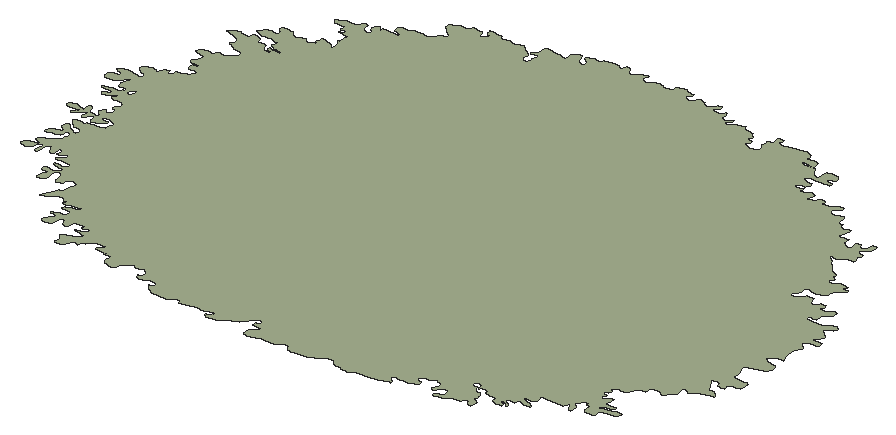
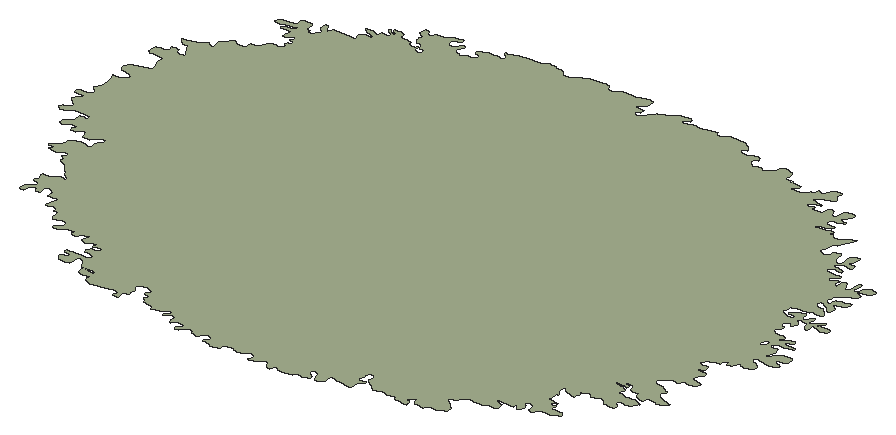
# SketchUp Ruby script. Lengths in inches.
U = 1.inch
M = Sketchup.active_model
def pt(a) = Geom::Point3d.new(a.map { |v| v * U })
def face(e, loops, mat)
  f = e.add_face(loops[0].map { |a| pt(a) })
  loops[1..].each { |l| e.add_face(l.map { |a| pt(a) }).erase! }
  f.material = f.back_material = mat if mat
  f
end
# faces: each face lists its corners as indices into pts; further lists are holes
def faces(e, pts, list, mat = nil) = list.each { |f| face(e, (f[0].is_a?(Array) ? f : [f]).map { |l| l.map { |i| pts[i] } }, mat) }
# xy, xz, yz: faces in a plane at the given z, y or x. An outline is a flat list of corners, or four numbers for a rectangle; further outlines are holes
def ring(l) = l.size == 4 ? [[l[0], l[1]], [l[2], l[1]], [l[2], l[3]], [l[0], l[3]]] : l.each_slice(2).to_a
def flat(e, list, mat, &to3) = list.each { |f| face(e, (f[0].is_a?(Array) ? f : [f]).map { |l| ring(l).map { |u, v| to3.(u, v) } }, mat) }
def xy(e, z, list, mat = nil) = flat(e, list, mat) { |x, y| [x, y, z] }
def xz(e, y, list, mat = nil) = flat(e, list, mat) { |x, z| [x, y, z] }
def yz(e, x, list, mat = nil) = flat(e, list, mat) { |y, z| [x, y, z] }
def lines(e, pts, list) = list.each { |a, b| e.add_line(pt(pts[a]), pt(pts[b])) }
# prism: a flat outline (further loops are holes) pulled along v
def prism(e, loops, v, mat = nil)
  f = face(e, loops, mat); d = Geom::Vector3d.new(v.map { |x| x * U })
  f.pushpull(f.normal.samedirection?(d) ? d.length : -d.length)
end
def box(e, o, s, mat = nil) = prism(e, [[o, [o[0] + s[0], o[1], o[2]], [o[0] + s[0], o[1] + s[1], o[2]], [o[0], o[1] + s[1], o[2]]]], [0, 0, s[2]], mat)
def at(x, y, z, deg = 0) = Geom::Transformation.translation(pt([x, y, z])) * Geom::Transformation.rotation(ORIGIN, Z_AXIS, deg.degrees)
def axes(o, x, y, z) = Geom::Transformation.new([*x, 0, *y, 0, *z, 0, *pt(o).to_a, 1])
def part(name) = M.definitions.add(name)
# library, detail: a bought-in or finely detailed component or shape, given as its bounding box
def library(name, o, s) = part(name).tap { |d| box(d.entities, o, s) }
def detail(e, o, s) = box(e.add_group.entities, o, s)
def put(e, d, t, mat = nil) = e.add_instance(d, t).tap { |i| i.material = mat if mat }
def group(e, t, mat = nil) = e.add_group.tap { |g| g.transformation = t; g.material = mat if mat }.entities
root = M.entities
M.materials.add("Boxwoodplan").color = [166, 177, 144]
xy(root,9,[[[264.536,68.149,264.425,68.153,264.33,68.178,264.274,68.234,264.272,68.337,264.298,68.401,264.362,68.464,264.411,68.528,264.469,68.625,264.283,68.655,264.193,68.664,264.213,68.752,264.299,68.81,264.33,68.82,264.325,68.865,264.236,68.897,264.12,68.856,264.023,68.726,263.88,68.571,263.719,68.484,263.614,68.461,263.553,68.436,263.537,68.393,263.393,68.301,263.199,68.271,263.11,68.279,263.03,68.326,263.03,68.347,263.075,68.378,263.166,68.456,263.234,68.503,263.145,68.517,263.032,68.5,262.912,68.455,262.816,68.464,262.719,68.474,262.622,68.466,262.495,68.422,262.295,68.376,262.206,68.369,262.168,68.462,262.16,68.484,262.093,68.492,262.004,68.474,261.835,68.356,261.636,68.347,261.405,68.373,261.238,68.466,261.097,68.63,261.28,68.722,261.18,68.775,261.044,68.792,260.918,68.769,260.846,68.716,260.765,68.692,260.649,68.757,260.607,68.825,260.695,68.866,260.722,68.927,260.726,68.977,260.685,69.029,260.613,69.105,260.527,69.137,260.44,69.084,260.374,69.058,260.318,69.1,260.301,69.123,260.277,69.141,260.248,69.131,260.169,69.077,260.097,69.029,260.021,68.943,260.009,68.81,259.938,68.768,259.888,68.743,259.828,68.745,259.729,68.765,259.642,68.813,259.598,68.881,259.59,68.971,259.599,69.037,259.612,69.059,259.593,69.1,259.379,69.119,259.447,69.155,259.421,69.156,259.328,69.15,259.159,69.166,259.082,69.192,259.064,69.226,259.079,69.244,259.204,69.333,259.202,69.39,259.117,69.413,258.958,69.409,258.827,69.339,258.73,69.253,258.655,69.218,258.608,69.192,258.607,69.173,258.643,69.121,258.627,69.066,258.557,69.101,258.493,69.14,258.432,69.092,258.41,69.037,258.378,68.923,258.331,68.875,258.258,68.841,258.167,68.836,258.097,68.861,258.078,68.894,258.085,68.912,258.106,68.952,258.128,69.011,258.097,69.068,257.996,69.169,258.11,69.249,258.171,69.289,258.251,69.304,258.318,69.335,258.373,69.389,258.458,69.496,258.386,69.522,258.307,69.53,258.174,69.55,258.136,69.585,258.143,69.604,258.218,69.639,258.38,69.677,258.422,69.728,258.417,69.768,258.391,69.783,258.241,69.731,258.195,69.752,258.196,69.771,258.219,69.834,258.058,69.845,257.977,69.853,257.923,69.845,257.916,69.826,257.9,69.729,257.885,69.662,257.843,69.611,257.796,69.598,257.777,69.613,257.718,69.659,257.673,69.777,257.634,69.803,257.607,69.804,257.553,69.796,257.546,69.777,257.544,69.661,257.49,69.543,257.429,69.469,257.349,69.439,257.27,69.442,257.224,69.467,257.191,69.526,257.191,69.583,257.245,69.697,257.359,69.804,257.379,69.822,257.366,69.843,257.339,69.848,257.259,69.866,257.178,69.879,257.151,69.895,257.158,69.914,257.178,69.933,257.327,70.001,257.489,70.025,257.531,70.127,257.505,70.188,257.457,70.21,257.43,70.206,257.267,70.188,257.226,70.219,257.233,70.239,257.26,70.299,257.418,70.353,257.59,70.423,257.638,70.462,257.625,70.483,257.529,70.456,257.357,70.437,257.213,70.392,257.124,70.405,257.097,70.411,257.103,70.431,257.124,70.446,257.179,70.49,257.151,70.527,257.124,70.523,257.041,70.531,256.986,70.579,256.972,70.621,256.945,70.617,256.862,70.594,256.705,70.508,256.556,70.432,256.482,70.4,256.427,70.412,256.44,70.432,256.459,70.472,256.486,70.489,256.51,70.569,256.56,70.67,256.592,70.778,256.643,70.832,256.717,70.871,256.76,70.992,256.782,71.132,256.802,71.246,256.798,71.305,256.753,71.341,256.672,71.354,256.586,71.354,256.512,71.33,256.503,71.265,256.503,71.203,256.47,71.144,256.382,71.107,256.325,71.116,256.287,71.175,256.276,71.236,256.25,71.357,256.245,71.419,256.204,71.473,256.177,71.495,256.139,71.51,256.081,71.499,256.046,71.479,256.044,71.448,256.036,71.386,256.039,71.249,256.064,71.187,256.056,71.123,256.005,71.058,255.957,71.03,255.919,71.018,255.881,71.023,255.839,71.031,255.821,71.058,255.817,71.186,255.838,71.243,255.884,71.296,255.899,71.326,255.891,71.354,255.834,71.359,255.752,71.366,255.715,71.381,255.692,71.41,255.689,71.472,255.704,71.503,255.739,71.519,255.911,71.491,255.99,71.516,256.039,71.546,256.1,71.593,256.113,71.656,256.09,71.682,256.046,71.683,255.969,71.69,255.877,71.701,255.776,71.737,255.757,71.766,255.763,71.78,255.782,71.783,255.842,71.795,256.017,71.781,256.107,71.806,256.119,71.864,256.093,71.926,256.021,71.966,255.943,71.972,255.829,71.966,255.729,71.94,255.646,71.958,255.642,71.988,255.663,72.016,255.709,72.073,255.775,72.13,255.828,72.21,255.82,72.244,255.775,72.261,255.71,72.259,255.592,72.159,255.553,72.161,255.518,72.181,255.54,72.24,255.556,72.307,255.513,72.369,255.473,72.386,255.453,72.387,255.447,72.372,255.451,72.326,255.449,72.184,255.408,72.122,255.368,72.127,255.333,72.151,255.235,72.282,255.211,72.347,255.186,72.374,255.171,72.363,255.116,72.3125,255.08,72.254,255.1,72.123,255.105,72.056,255.085,71.991,255.035,71.982,255.001,71.998,254.991,72.042,255.011,72.174,255.02,72.252,255.02,72.29,255.005,72.302,254.99,72.291,254.911,72.257,254.871,72.202,254.862,72.139,254.823,72.097,254.686,72.006,254.646,71.997,254.602,72.006,254.522,72.046,254.502,72.076,254.506,72.109,254.539,72.17,254.637,72.256,254.726,72.283,254.816,72.283,254.911,72.287,254.85,72.338,254.699,72.424,254.683,72.485,254.735,72.523,254.827,72.593,254.946,72.654,255.064,72.729,255.1,72.742,255.126,72.766,255.152,72.809,255.155,72.901,255.1875,73.022,255.189,73.084,255.168,73.105,255.146,73.114,255.083,73.129,255.05,73.124,255.046,73.108,255.058,73.015,255.016,72.954,254.968,72.918,254.891,72.89,254.82,72.878,254.659,72.853,254.624,72.858,254.611,72.872,254.611,72.88,254.62,72.92,254.637,72.967,254.679,73.014,254.748,73.061,254.807,73.083,254.865,73.085,254.904,73.087,254.924,73.095,254.947,73.116,254.942,73.14,254.888,73.171,254.82,73.227,254.788,73.284,254.784,73.351,254.797,73.401,254.849,73.446,254.875,73.451,254.886,73.445,254.906,73.431,254.949,73.37,254.998,73.324,255.126,73.246,255.2,73.212,255.235,73.196,255.255,73.204,255.279,73.226,255.286,73.242,255.297,73.283,255.282,73.34,255.239,73.386,255.207,73.409,255.173,73.421,255.113,73.421,255.039,73.424,254.996,73.466,254.91,73.538,254.851,73.589,254.812,73.636,254.813,73.665,254.837,73.691,254.893,73.718,254.928,73.723,254.969,73.719,255.03,73.699,255.091,73.697,255.127,73.704,255.161,73.745,255.21,73.777,255.27,73.784,255.34,73.783,255.494,73.791,255.634,73.811,255.667,73.828,255.668,73.846,255.662,73.888,255.65,73.932,255.662,73.976,255.691,74.08,255.678,74.103,255.655,74.116,255.599,74.146,255.545,74.183,255.473,74.211,255.399,74.214,255.349,74.204,255.328,74.19,255.303,74.138,255.308,74.117,255.319,74.113,255.343,74.108,255.494,74.096,255.52,74.091,255.525,74.082,255.516,74.066,255.476,74.026,255.431,73.983,255.366,73.947,255.304,73.904,255.232,73.868,255.195,73.872,255.175,73.883,255.15,73.92,255.143,74.015,255.126,74.04,255.144,74.054,255.15,74.097,255.145,74.107,255.133,74.108,255.118,74.106,255.092,74.103,255.06,74.096,255.042,74.084,254.961,73.989,254.929,73.934,254.898,73.911,254.875,73.914,254.849,73.935,254.841,73.952,254.834,73.992,254.863,74.077,254.868,74.122,254.859,74.149,254.839,74.156,254.801,74.147,254.781,74.134,254.735,74.084,254.613,73.977,254.577,73.952,254.551,73.947,254.514,73.954,254.502,73.971,254.593,74.077,254.656,74.122,254.67,74.148,254.669,74.165,254.661,74.172,254.649,74.168,254.634,74.162,254.603,74.151,254.519,74.127,254.352,74.109,254.279,74.116,254.231,74.141,254.209,74.168,254.208,74.185,254.225,74.237,254.273,74.283,254.333,74.3,254.404,74.304,254.478,74.286,254.606,74.243,254.692,74.217,254.703,74.22,254.703,74.239,254.694,74.259,254.669,74.306,254.668,74.362,254.675,74.427,254.687,74.457,254.704,74.469,254.753,74.432,254.792,74.383,254.819,74.337,254.829,74.275,254.841,74.223,254.856,74.195,254.879,74.195,255.014,74.177,255.087,74.163,255.122,74.16,255.14,74.174,255.155,74.222,255.1,74.264,255.042,74.328,255.024,74.355,255.024,74.372,255.058,74.48,255.088,74.503,255.115,74.508,255.13,74.497,255.139,74.479,255.168,74.434,255.179,74.409,255.191,74.411,255.213,74.423,255.292,74.501,255.309,74.547,255.31,74.599,255.296,74.631,255.275,74.643,255.212,74.666,255.172,74.685,255.164,74.706,255.18,74.756,255.236,74.793,255.27,74.815,255.283,74.835,255.291,74.889,255.289,74.936,255.194,75.011,255.05,75.034,254.988,75.05,254.953,75.033,254.925,75.034,254.856,75.051,254.837,75.078,254.846,75.102,254.972,75.204,254.966,75.237,254.944,75.252,254.899,75.244,254.871,75.235,254.744,75.174,254.704,75.127,254.655,75.083,254.586,75.068,254.558,75.069,254.511,75.121,254.539,75.146,254.557,75.185,254.588,75.208,254.682,75.239,254.727,75.269,254.716,75.3,254.703,75.303,254.693,75.296,254.667,75.289,254.628,75.292,254.493,75.304,254.346,75.332,254.322,75.347,254.328,75.366,254.353,75.395,254.566,75.455,254.629,75.454,254.69,75.438,254.75,75.41,254.777,75.412,254.783,75.422,254.832,75.5,254.856,75.515,254.862,75.534,254.862,75.602,254.852,75.613,254.838,75.61,254.78,75.611,254.723,75.604,254.676,75.587,254.652,75.595,254.631,75.616,254.606,75.649,254.586,75.737,254.597,75.826,254.627,75.868,254.633,75.9,254.646,75.942,254.684,75.964,254.679,76.01,254.657,76.046,254.568,76.023,254.55,75.989,254.551,75.969,254.554,75.906,254.474,75.859,254.333,75.765,254.177,75.72,254.093,75.745,254.051,75.798,254.042,75.924,254.17,76.009,254.253,76.023,254.297,76.047,254.32,76.081,254.319,76.101,254.233,76.132,254.16,76.158,254.098,76.214,254.133,76.268,254.209,76.297,254.305,76.331,254.37,76.33,254.549,76.287,254.641,76.265,254.726,76.269,254.777,76.289,254.783,76.309,254.767,76.375,254.706,76.427,254.661,76.434,254.549,76.505,254.502,76.547,254.488,76.583,254.481,76.637,254.481,76.664,254.494,76.679,254.536,76.714,254.587,76.729,254.701,76.76,254.732,76.77,254.772,76.77,254.822,76.765,254.835,76.753,254.85,76.723,254.864,76.709,254.874,76.709,254.902,76.712,254.918,76.724,254.939,76.774,254.967,76.807,254.983,76.83,254.986,76.855,255.002,76.88,255.022,76.892,255.07,76.904,255.109,76.896,255.13,76.853,255.135,76.801,255.151,76.774,255.172,76.774,255.214,76.816,255.239,76.858,255.254,76.962,255.269,76.987,255.301,76.994,255.333,76.994,255.352,76.982,255.373,76.96,255.405,76.959,255.458,76.981,255.502,77.027,255.516,77.051,255.505,77.065,255.565,77.063,255.594,77.066,255.61,77.085,255.615,77.134,255.649,77.174,255.683,77.22,255.629,77.263,255.562,77.292,255.525,77.291,255.492,77.28,255.45,77.269,255.408,77.275,255.386,77.291,255.365,77.314,255.342,77.417,255.355,77.442,255.36,77.459,255.371,77.462,255.475,77.483,255.521,77.491,255.539,77.502,255.529,77.506,255.444,77.534,255.378,77.546,255.349,77.539,255.314,77.539,255.278,77.54,255.242,77.552,255.204,77.602,255.186,77.631,255.186,77.662,255.201,77.683,255.23,77.698,255.261,77.717,255.27,77.744,255.326,77.856,255.332,77.909,255.325,77.936,255.285,77.947,255.207,77.973,255.034,78.02,254.998,78.038,254.981,78.062,255.017,78.116,255.061,78.151,255.107,78.178,255.162,78.198,255.214,78.207,255.267,78.204,255.322,78.18,255.377,78.182,255.404,78.186,255.417,78.207,255.434,78.248,255.472,78.284,255.492,78.302,255.518,78.304,255.587,78.287,255.649,78.276,255.676,78.273,255.699,78.288,255.786,78.355,255.873,78.421,255.927,78.517,255.923,78.562,255.882,78.598,255.765,78.636,255.639,78.667,255.553,78.739,255.495,78.774,255.426,78.795,255.399,78.807,255.385,78.828,255.407,78.874,255.455,78.916,255.453,79.001,255.403,79.079,255.273,79.136,254.985,79.232,254.964,79.266,255.036,79.33,255.157,79.382,255.262,79.386,255.319,79.373,255.364,79.347,255.412,79.337,255.465,79.345,255.526,79.357,255.555,79.388,255.57,79.467,255.587,79.502,255.641,79.501,255.698,79.491,255.746,79.471,255.813,79.412,255.837,79.377,255.851,79.337,255.852,79.269,255.859,79.264,255.867,79.269,255.894,79.282,255.945,79.288,256.034,79.29,256.114,79.254,256.148,79.19,256.173,79.112,256.243,79.067,256.283,79.054,256.301,79.054,256.328,79.063,256.423,79.069,256.44,79.074,256.42,79.091,256.357,79.114,256.305,79.119,256.267,79.137,256.248,79.172,256.245,79.184,256.249,79.204,256.263,79.211,256.298,79.211,256.34,79.204,256.446,79.176,256.561,79.171,256.613,79.179,256.631,79.181,256.658,79.193,256.613,79.223,256.572,79.233,256.486,79.247,256.428,79.261,256.387,79.264,256.365,79.268,256.34,79.282,256.288,79.309,256.241,79.335,256.219,79.367,256.229,79.423,256.258,79.462,256.299,79.491,256.259,79.522,256.204,79.537,256.161,79.54,256.106,79.548,256.075,79.574,256.057,79.611,256.043,79.62,256.014,79.619,255.899,79.591,255.846,79.577,255.797,79.578,255.75,79.581,255.7,79.598,255.652,79.615,255.612,79.622,255.569,79.646,255.526,79.669,255.551,79.682,255.553,79.689,255.564,79.729,255.58,79.765,255.606,79.802,255.637,79.834,255.681,79.859,255.734,79.881,255.779,79.893,255.885,79.887,255.962,79.881,255.996,79.877,256.006,79.877,256.006,79.89,255.998,79.932,255.977,79.976,255.941,80.015,255.898,80.046,255.865,80.092,255.867,80.116,255.878,80.136,255.925,80.166,255.978,80.189,256.004,80.189,256.03,80.183,256.084,80.167,256.152,80.162,256.199,80.147,256.223,80.134,256.241,80.115,256.285,80.074,256.324,80.04,256.369,80.008,256.425,79.995,256.479,80,256.524,80.029,256.556,80.065,256.605,80.103,256.631,80.103,256.653,80.088,256.694,80.047,256.741,80.013,256.869,80.038,256.943,80.057,256.985,80.085,256.99,80.105,256.969,80.121,256.918,80.143,256.908,80.166,256.916,80.189,256.932,80.233,256.939,80.293,256.943,80.318,256.966,80.334,256.993,80.336,257.023,80.327,257.065,80.308,257.199,80.268,257.26,80.246,257.299,80.213,257.326,80.173,257.341,80.15,257.348,80.142,257.357,80.146,257.365,80.151,257.398,80.196,257.404,80.231,257.394,80.334,257.372,80.382,257.348,80.417,257.313,80.456,257.303,80.485,257.314,80.497,257.325,80.494,257.347,80.496,257.346,80.504,257.351,80.527,257.344,80.569,257.329,80.725,257.331,80.802,257.216,80.821,257.119,80.824,257.057,80.832,257.039,80.839,257.025,80.849,257.038,80.859,257.151,80.901,257.185,80.93,257.184,80.943,257.161,80.967,257.125,80.971,257.072,80.96,257.024,80.938,257.007,80.938,256.992,80.965,257.019,81.048,257.021,81.088,257.02,81.102,256.996,81.123,256.907,81.105,256.794,81.108,256.685,81.124,256.624,81.205,256.622,81.232,256.66,81.269,256.756,81.323,256.805,81.349,256.859,81.355,256.984,81.352,257.075,81.356,257.135,81.365,257.175,81.403,257.215,81.438,257.223,81.481,257.249,81.52,257.305,81.533,257.342,81.528,257.385,81.494,257.396,81.408,257.403,81.319,257.427,81.277,257.482,81.251,257.574,81.231,257.629,81.254,257.647,81.295,257.624,81.338,257.577,81.375,257.521,81.462,257.557,81.541,257.631,81.623,257.65,81.626,257.674,81.596,257.693,81.548,257.767,81.466,257.795,81.44,257.786,81.495,257.768,81.59,257.824,81.607,257.885,81.601,258.012,81.598,258.125,81.595,258.247,81.577,258.265,81.577,258.253,81.606,258.202,81.648,258.072,81.7,258.034,81.709,258.011,81.754,258.013,81.845,258.048,81.89,258.097,81.916,258.213,81.921,258.31,81.93,258.405,81.997,258.531,82.001,258.647,81.991,258.743,81.972,258.864,81.965,258.907,82.011,258.921,82.058,258.963,82.152,259.052,82.206,259.172,82.264,259.184,82.28,259.167,82.313,259.127,82.351,259.019,82.433,258.951,82.506,258.893,82.548,258.836,82.59,258.867,82.597,258.866,82.61,258.861,82.631,258.85,82.699,258.853,82.729,258.888,82.764,258.971,82.804,259.054,82.841,259.092,82.847,259.148,82.845,259.235,82.836,259.259,82.828,259.282,82.83,259.314,82.863,259.366,82.938,259.402,82.952,259.459,82.955,259.561,82.95,259.657,82.918,259.689,82.897,259.718,82.855,259.719,82.784,259.722,82.756,259.727,82.734,259.75,82.724,259.803,82.734,259.848,82.764,259.91,82.818,259.935,82.841,259.956,82.853,259.969,82.87,259.885,82.917,259.846,82.932,259.803,82.976,259.778,83.055,259.779,83.086,259.837,83.103,260.029,83.074,260.126,83.059,260.161,83.045,260.161,82.999,260.171,82.971,260.231,82.967,260.335,82.982,260.437,82.995,260.479,82.991,260.526,82.977,260.553,82.954,260.578,82.953,260.603,82.962,260.747,82.991,260.788,83,260.84,83.007,260.876,83.003,260.921,82.977,260.951,82.906,260.977,82.882,261.022,82.864,261.062,82.853,261.102,82.828,261.154,82.773,261.208,82.716,261.195,82.639,261.188,82.565,261.202,82.535,261.233,82.504,261.26,82.481,261.307,82.473,261.344,82.47,261.388,82.5,261.401,82.532,261.402,82.573,261.39,82.647,261.427,82.807,261.416,82.836,261.398,82.849,261.374,82.852,261.335,82.853,261.283,82.847,261.247,82.846,261.201,82.854,261.175,82.877,261.182,82.899,261.21,82.916,261.249,82.93,261.294,82.957,261.319,83.032,261.323,83.197,261.323,83.229,261.346,83.248,261.372,83.252,261.471,83.242,261.67,83.22,261.761,83.21,261.85,83.189,261.937,83.173,261.988,83.166,261.983,83.374,262.051,83.446,262.136,83.506,262.19,83.496,262.218,83.461,262.266,83.39,262.289,83.316,262.297,83.28,262.295,83.261,262.322,83.226,262.427,83.193,262.479,83.193,262.518,83.224,262.521,83.299,262.418,83.379,262.34,83.438,262.352,83.473,262.396,83.509,262.49,83.56,262.54,83.569,262.621,83.557,262.725,83.557,262.748,83.635,262.958,83.663,263.058,83.681,263.166,83.667,263.245,83.598,263.278,83.563,263.305,83.56,263.345,83.588,263.343,83.663,263.334,83.705,263.347,83.739,263.397,83.749,263.452,83.734,263.523,83.641,263.544,83.567,263.577,83.532,263.626,83.518,263.677,83.522,263.723,83.55,263.811,83.633,263.892,83.6875,263.994,83.734,264.042,83.719,264.056,83.683,264.004,83.612,263.978,83.577,263.986,83.535,264.075,83.477,264.175,83.462,264.225,83.471,264.275,83.518,264.353,83.586,264.468,83.601,264.583,83.573,264.614,83.543,264.691,83.512,264.791,83.53,264.873,83.584,264.873,83.697,264.93,83.74,265.043,83.764,265.148,83.759,265.229,83.7,265.375,83.68,265.429,83.67,265.435,83.633,265.361,83.566,265.328,83.493,265.341,83.456,265.412,83.416,265.514,83.42,265.567,83.453,265.587,83.492,265.608,83.564,265.656,83.587,265.68,83.598,265.731,83.598,265.834,83.56,265.877,83.489,265.963,83.436,266.094,83.466,266.128,83.497,266.134,83.54,266.174,83.623,266.281,83.641,266.311,83.611,266.317,83.57,266.265,83.486,266.216,83.468,266.189,83.433,266.25,83.368,266.38,83.356,266.471,83.392,266.538,83.463,266.563,83.47,266.572,83.452,266.59,83.412,266.614,83.377,266.603,83.32,266.583,83.277,266.601,83.242,266.69,83.199,266.798,83.204,266.853,83.222,266.904,83.277,266.921,83.293,266.923,83.274,266.91,83.232,266.837,83.152,266.803,83.121,266.814,83.086,266.862,83.067,266.919,83.067,267.015,83.108,267.097,83.165,267.317,83.244,267.339,83.173,267.362,83.143,267.413,83.138,267.529,83.13,267.653,83.104,267.668,83.032,267.691,83.002,267.737,82.984,267.76,82.949,267.746,82.912,267.719,82.814,267.836,82.793,267.882,82.774,267.892,82.739,267.818,82.67,267.804,82.633,267.82,82.598,267.896,82.547,267.999,82.52,268.1,82.515,268.212,82.583,268.254,82.658,268.196,82.73,268.163,82.799,268.183,82.905,268.192,82.942,268.163,82.975,268.159,83.011,268.201,83.038,268.302,83.042,268.291,83.141,268.249,83.293,268.299,83.307,268.364,83.294,268.417,83.276,268.448,83.219,268.398,83.151,268.402,83.115,268.448,83.096,268.556,83.096,268.686,83.13,269.193,83.197,269.239,83.1875,269.285,83.164,269.331,83.141,269.365,83.117,269.396,83.047,269.379,82.955,269.583,82.969,269.648,82.962,269.733,82.931,269.77,82.824,269.755,82.777,269.739,82.744,269.698,82.737,269.528,82.768,269.464,82.774,269.421,82.775,269.401,82.769,269.398,82.753,269.426,82.705,269.467,82.685,269.514,82.686,269.687,82.701,269.756,82.703,269.84,82.668,269.878,82.628,269.908,82.566,269.976,82.456,270.055,82.417,270.14,82.413,270.171,82.454,270.165,82.538,270.147,82.59,270.154,82.656,270.195,82.706,270.296,82.738,270.405,82.752,270.494,82.721,270.542,82.679,270.576,82.616,270.577,82.57,270.515,82.515,270.449,82.502,270.408,82.49,270.376,82.457,270.38,82.427,270.429,82.408,270.527,82.382,270.598,82.358,270.618,82.326,270.606,82.294,270.552,82.267,270.465,82.259,270.303,82.253,270.216,82.241,270.127,82.275,270.0625,82.289,269.981,82.27,269.925,82.227,269.923,82.163,269.982,82.123,270.068,82.1,270.154,82.085,270.201,82.086,270.235,82.066,270.256,82.023,270.239,81.958,270.204,81.91,270.176,81.885,270.131,81.874,269.989,81.854,269.969,81.849,269.966,81.833,269.96,81.803,269.965,81.77,270.009,81.752,270.076,81.75,270.118,81.75,270.167,81.766,270.23,81.797,270.244,81.732,270.215,81.685,270.208,81.655,270.247,81.636,270.308,81.642,270.39,81.689,270.446,81.731,270.474,81.756,270.512,81.74,270.576,81.724,270.645,81.671,270.641,81.623,270.598,81.557,270.565,81.492,270.584,81.468,270.63,81.465,270.706,81.475,270.788,81.515,270.827,81.573,270.899,81.616,270.959,81.629,270.996,81.621,271.014,81.597,271.018,81.568,271,81.541,270.972,81.517,270.974,81.502,270.995,81.5,271.167,81.519,271.248,81.53,271.315,81.572,271.357,81.609,271.436,81.634,271.533,81.639,271.556,81.615,271.559,81.586,271.399,81.369,271.414,81.323,271.471,81.271,271.554,81.256,271.643,81.275,271.711,81.302,271.796,81.324,271.861,81.233,271.897,81.019,271.899,81.005,271.935,80.994,272.019,81.015,272.03,80.938,272.054,80.89,272.13,80.881,272.267,80.915,272.335,80.913,272.35,80.859,272.282,80.638,272.271,80.587,272.294,80.534,272.36,80.505,272.428,80.516,272.564,80.543,272.584,80.438,272.579,80.336,272.701,80.267,272.834,80.236,272.864,80.337,272.854,80.441,272.831,80.493,272.86,80.544,272.928,80.555,272.967,80.501,272.989,80.448,273.037,80.414,273.114,80.437,273.168,80.487,273.192,80.603,273.196,80.655,273.257,80.679,273.314,80.651,273.344,80.597,273.319,80.474,273.204,80.395,273.151,80.358,273.131,80.301,273.11,80.251,273.133,80.205,273.265,80.181,273.321,80.153,273.326,80.102,273.253,80.017,273.288,79.915,273.317,79.863,273.305,79.814,273.171,79.788,273.07,79.748,272.966,79.678,272.915,79.643,272.849,79.645,272.785,79.679,272.753,79.686,272.727,79.663,272.771,79.569,272.89,79.503,272.937,79.464,272.934,79.415,273.019,79.339,273.185,79.152,273.317,79.069,273.38,79.055,273.418,79.012,273.402,78.917,273.518,78.854,273.455,78.768,273.435,78.716,273.433,78.693,273.464,78.68,273.602,78.698,273.736,78.775,273.866,78.787,273.991,78.753,273.995,78.706,273.928,78.68,273.902,78.663,273.916,78.639,273.994,78.619,274.066,78.616,274.098,78.615,274.111,78.591,274.023,78.502,273.857,78.342,273.833,78.251,273.829,78.206,273.801,78.162,273.708,78.087,273.58,78.058,273.455,78.063,273.346,78.102,273.277,78.096,273.25,78.024,273.277,77.914,273.248,77.807,273.13,77.74,273.158,77.64,273.296,77.661,273.468,77.852,273.695,77.835,273.771,77.625,273.816,77.614,273.898,77.638,273.985,77.742,274.123,77.755,274.161,77.655,274.111,77.594,274.096,77.559,274.173,77.52,274.312,77.551,274.431,77.617,274.478,77.633,274.568,77.612,274.546,77.497,274.435,77.403,274.371,77.309,274.378,77.132,274.364,77.098,274.272,77.075,274.139,77.107,274.164,77.001,274.296,76.961,274.441,76.955,274.59,76.984,274.827,77.106,274.963,77.118,275.055,77.027,275.022,76.924,274.882,76.869,274.835,76.845,274.807,76.785,274.91,76.695,275.061,76.535,275.028,76.434,274.912,76.379,274.876,76.355,274.914,76.294,275.058,76.288,275.188,76.266,275.2,76.165,275.127,76.109,274.994,76.097,274.869,76.06,274.826,75.962,274.994,75.781,274.887,75.588,274.89,75.408,274.944,75.195,274.988,75.097,274.856,75.07,274.733,75.027,274.639,74.951,274.612,74.889,274.723,74.821,274.975,74.764,275.052,74.682,275.073,74.579,275.031,74.487,274.916,74.413,274.455,74.253,274.457,74.161,274.501,74.067,274.555,73.974,274.556,73.883,274.551,73.822,274.548,73.792,274.574,73.738,274.695,73.696,274.82,73.691,274.946,73.701,274.988,73.7,275.046,73.652,275.057,73.473,275.03,73.414,274.921,73.367,274.795,73.349,274.753,73.351,274.707,73.301,274.749,73.211,274.736,73.182,274.651,73.163,274.61,73.165,274.54,73.19,274.508,73.279,274.439,73.311,274.315,73.316,274.273,73.31,274.257,73.252,274.333,73.176,274.42,73.012,274.449,72.989,274.474,72.937,274.492,72.907,274.573,72.897,274.653,72.879,274.738,72.811,274.801,72.73,274.798,72.701,274.714,72.676,274.465,72.635,274.27,72.508,274.197,72.489,274.102,72.564,274.0625,72.572,273.998,72.539,274.001,72.454,274.057,72.29,274.015,72.283,273.982,72.239,273.933,72.199,273.879,72.086,273.84,72.038,273.806,72.019,273.77,72.033,273.648,72.119,273.585,72.134,273.543,72.136,273.497,72.117,273.434,72.083,273.404,72.01,273.414,71.957,273.396,71.894,273.234,71.872,273.182,71.83,273.15,71.779,273.103,71.737,273.091,71.675,273.06,71.629,273.026,71.603,272.989,71.592,272.92,71.583,272.822,71.595,272.762,71.57,272.7,71.522,272.67,71.477,272.745,71.439,272.772,71.396,272.736,71.34,272.681,71.304,272.66,71.244,272.658,71.214,272.678,71.206,272.749,71.199,272.775,71.202,272.795,71.201,272.799,71.186,272.761,71.116,272.742,71.069,272.739,71.039,272.78,71.038,272.92,71.114,272.988,71.13,273.069,71.127,273.053,71.023,273.036,70.91,273.035,70.862,273.058,70.84,273.098,70.838,273.162,70.865,273.243,70.865,273.302,70.852,273.342,70.847,273.348,70.817,273.308,70.779,273.229,70.75,273.163,70.741,273.08,70.716,273.041,70.678,273.025,70.621,273.028,70.607,273.068,70.606,273.15,70.631,273.308,70.693,273.462,70.723,273.588,70.725,273.64,70.705,273.615,70.631,273.594,70.589,273.533,70.538,273.38,70.512,273.241,70.51,273.18,70.502,273.149,70.447,273.175,70.328,273.16,70.283,273.079,70.262,272.943,70.275,272.885,70.28,272.841,70.334,272.832,70.445,272.832,70.487,272.82,70.516,272.811,70.531,272.791,70.531,272.733,70.544,272.728,70.601,272.73,70.615,272.726,70.629,272.707,70.634,272.627,70.637,272.57,70.611,272.526,70.556,272.488,70.518,272.463,70.46,272.474,70.41,272.53,70.374,272.605,70.274,272.601,70.175,272.592,70.135,272.585,70.108,272.554,70.085,272.535,70.086,272.513,70.117,272.484,70.176,272.419,70.278,272.378,70.317,272.364,70.332,272.354,70.318,272.347,70.291,272.343,70.246,272.324,70.193,272.319,70.179,272.288,70.163,272.205,70.156,272.064,70.159,271.778,70.16,271.72,70.182,271.633,70.192,271.614,70.183,271.608,70.153,271.658,70.093,271.683,69.995,271.677,69.956,271.645,69.916,271.621,69.909,271.561,69.9,271.458,69.9,271.36,69.904,271.312,69.872,271.367,69.848,271.468,69.833,271.576,69.8,271.651,69.746,271.732,69.673,271.714,69.649,271.653,69.633,271.552,69.641,271.515,69.649,271.464,69.669,271.416,69.704,271.366,69.728,271.331,69.649,271.321,69.578,271.281,69.565,271.225,69.578,271.18,69.608,271.167,69.62,271.149,69.628,271.137,69.61,271.103,69.533,271.105,69.504,271.138,69.467,271.23,69.436,271.269,69.402,271.282,69.36,271.28,69.346,271.261,69.343,271.218,69.38,271.138,69.429,271.045,69.446,270.988,69.449,270.976,69.435,270.997,69.409,271.111,69.366,271.148,69.354,271.171,69.312,271.168,69.284,271.166,69.27,271.123,69.268,271.01,69.28,270.905,69.315,270.87,69.344,270.861,69.39,270.86,69.461,270.809,69.48,270.75,69.461,270.65,69.469,270.551,69.487,270.525,69.509,270.499,69.545,270.503,69.588,270.509,69.602,270.472,69.611,270.377,69.636,270.339,69.637,270.32,69.638,270.285,69.625,270.273,69.597,270.253,69.591,270.226,69.617,270.223,69.631,270.254,69.655,270.269,69.665,270.261,69.691,270.174,69.748,270.137,69.772,270.118,69.776,270.077,69.756,270.037,69.736,270.017,69.729,270.006,69.701,270.029,69.61,270.125,69.606,270.163,69.601,270.193,69.561,270.186,69.533,270.18,69.519,270.188,69.49,270.3,69.454,270.387,69.416,270.448,69.357,270.465,69.332,270.464,69.318,270.429,69.302,270.409,69.293,270.44,69.271,270.495,69.244,270.507,69.22,270.456,69.1875,270.444,69.16,270.469,69.125,270.554,69.081,270.632,69.014,270.631,68.87,270.61,68.845,270.558,68.833,270.504,68.849,270.466,68.893,270.426,68.958,270.408,68.969,270.37,68.964,270.318,68.946,270.297,68.916,270.297,68.873,270.296,68.86,270.263,68.848,270.086,68.838,270.078,68.845,270.03,68.827,269.986,68.796,269.902,68.711,269.85,68.681,269.776,68.671,269.638,68.663,269.584,68.678,269.582,68.717,269.691,68.781,269.792,68.853,269.788,68.956,269.782,69,269.782,69.013,269.751,69.035,269.691,69.054,269.617,69.053,269.534,68.969,269.513,68.93,269.456,68.886,269.442,68.877,269.405,68.885,269.368,68.899,269.356,68.926,269.396,69.018,269.456,69.114,269.458,69.154,269.389,69.208,269.278,69.243,269.226,69.266,269.189,69.257,269.164,69.234,269.13,69.191,269.097,69.175,269.055,69.177,268.999,69.186,268.962,69.1875,268.924,69.165,268.843,69.07,268.857,69.029,268.931,68.99,268.986,68.957,269.013,68.936,269.022,68.91,268.998,68.871,268.938,68.827,268.836,68.775,268.781,68.755,268.708,68.758,268.653,68.779,268.58,68.789,268.534,68.764,268.497,68.762,268.465,68.78,268.41,68.785,268.337,68.772,268.315,68.737,268.325,68.679,268.422,68.595,268.449,68.555,268.45,68.53,268.45,68.517,268.432,68.511,268.142,68.411,267.867,68.389,267.634,68.392,267.543,68.39,267.421,68.329,267.318,68.295,267.221,68.299,267.184,68.3,267.134,68.319,267.086,68.348,267.025,68.345,266.936,68.354,266.852,68.395,266.792,68.452,266.761,68.498,266.703,68.511,266.603,68.498,266.507,68.458,266.427,68.417,266.328,68.344,266.231,68.288,266.138,68.259,265.897,68.241,265.707,68.206,265.61,68.209,265.545,68.304,265.514,68.37,265.426,68.385,265.335,68.372,265.239,68.3,265.174,68.237,265.084,68.23,264.907,68.253,264.722,68.26,264.644,68.209],[255.044,75.434,255.086,75.439,255.106,75.442,255.132,75.45,255.144,75.494,255.145,75.532,255.152,75.617,255.144,75.65,255.132,75.663,255.132,75.677,255.089,75.654,255.033,75.632,255.013,75.626,254.997,75.609,254.976,75.577,254.966,75.539,254.968,75.495,254.987,75.457,255.006,75.441]]],"Boxwoodplan")
